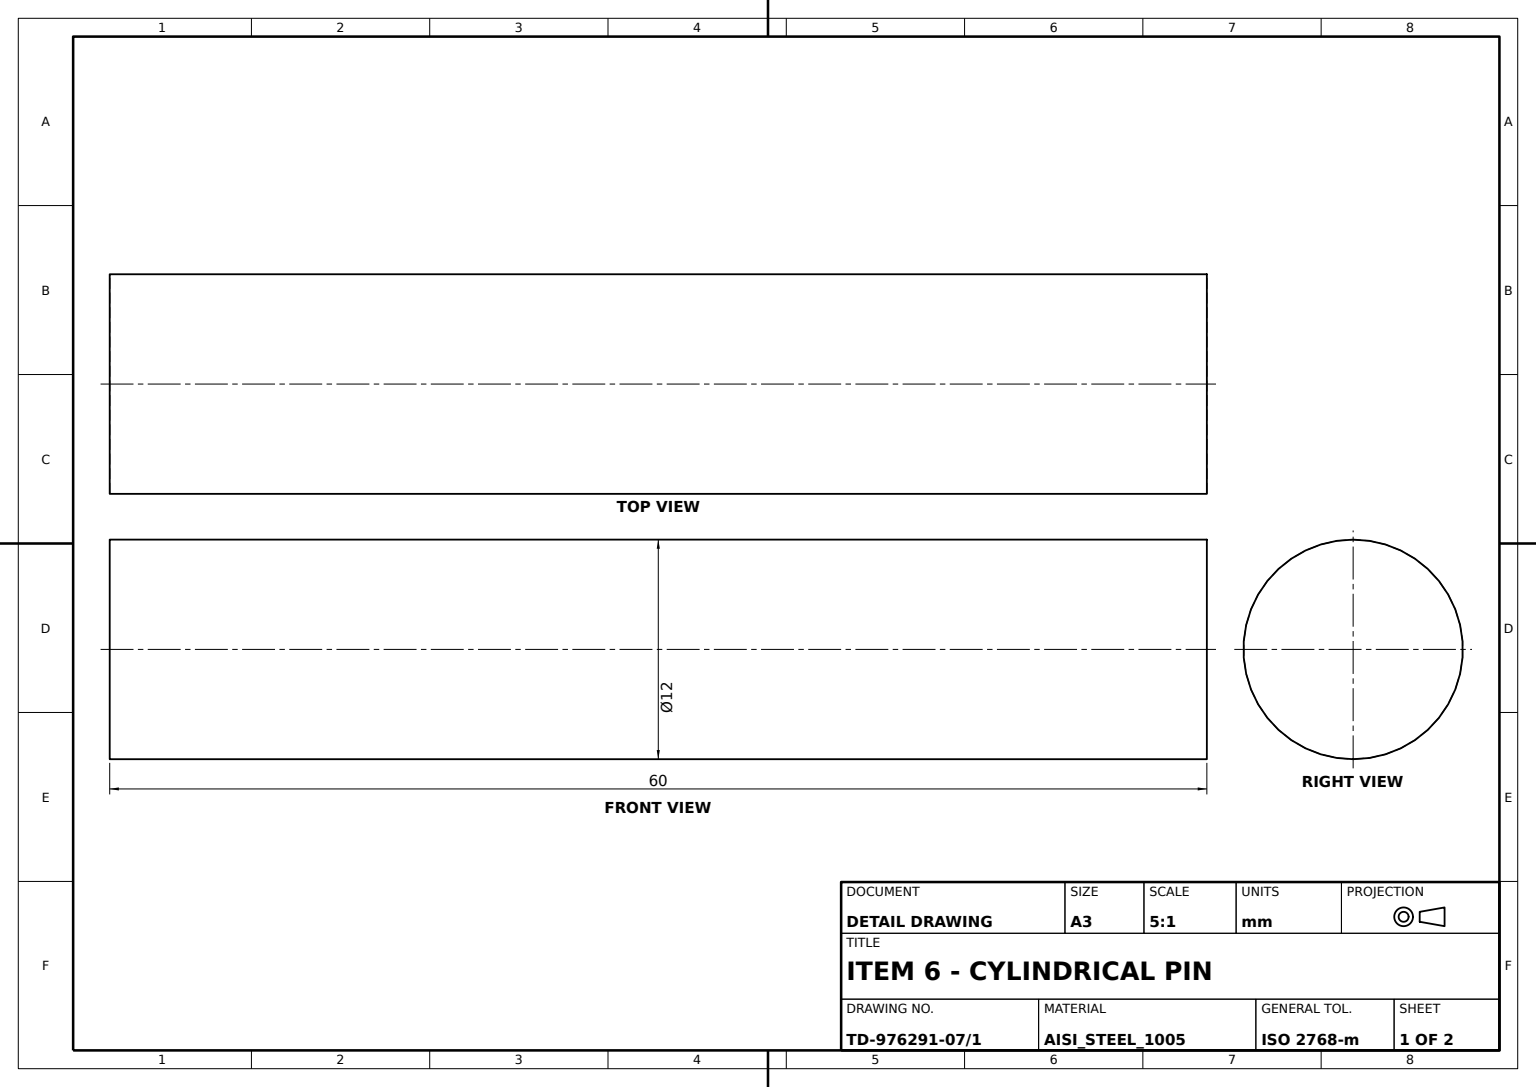
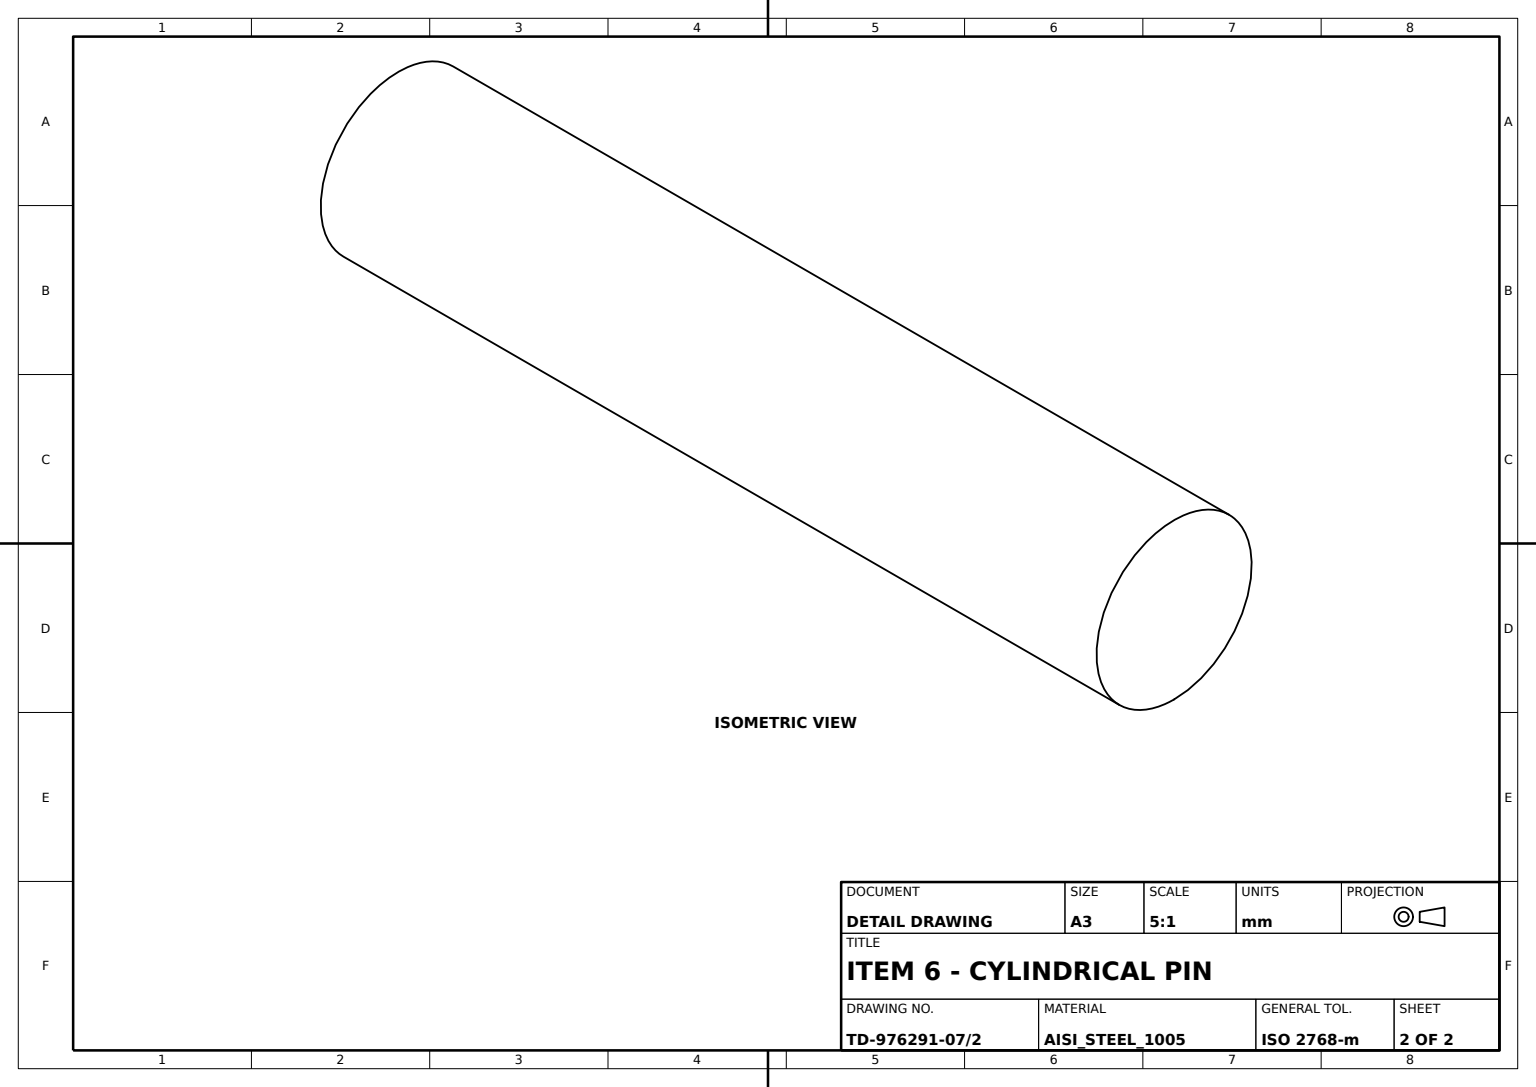
ISO-10303-21;
HEADER;
FILE_DESCRIPTION((''),'2;1');
FILE_NAME('','',(''),(''),'','','');
FILE_SCHEMA(('AUTOMOTIVE_DESIGN'));
ENDSEC;
DATA;
#1=APPLICATION_CONTEXT('');
#2=PRODUCT_CONTEXT('',#1,'mechanical');
#3=PRODUCT('','','',(#2));
#4=PRODUCT_DEFINITION_FORMATION('','',#3);
#5=PRODUCT_DEFINITION_CONTEXT('',#1,'design');
#6=PRODUCT_DEFINITION('','',#4,#5);
#7=PRODUCT_DEFINITION_SHAPE('','',#6);
#8=(LENGTH_UNIT()NAMED_UNIT(*)SI_UNIT(.MILLI.,.METRE.));
#9=(NAMED_UNIT(*)PLANE_ANGLE_UNIT()SI_UNIT($,.RADIAN.));
#10=(NAMED_UNIT(*)SI_UNIT($,.STERADIAN.)SOLID_ANGLE_UNIT());
#11=UNCERTAINTY_MEASURE_WITH_UNIT(LENGTH_MEASURE(0.005),#8,'distance_accuracy_value','');
#12=(GEOMETRIC_REPRESENTATION_CONTEXT(3)GLOBAL_UNCERTAINTY_ASSIGNED_CONTEXT((#11))GLOBAL_UNIT_ASSIGNED_CONTEXT((#8,#9,#10))REPRESENTATION_CONTEXT('',''));
#13=CARTESIAN_POINT('',(6.,0.,-30.));
#14=VERTEX_POINT('',#13);
#15=CARTESIAN_POINT('',(0.,0.,-30.));
#16=DIRECTION('',(0.,0.,1.));
#17=DIRECTION('',(1.,0.,0.));
#18=AXIS2_PLACEMENT_3D('',#15,#16,#17);
#19=CIRCLE('',#18,6.);
#20=EDGE_CURVE('',#14,#14,#19,.T.);
#21=ORIENTED_EDGE('',*,*,#20,.F.);
#22=EDGE_LOOP('',(#21));
#23=FACE_BOUND('',#22,.T.);
#24=PLANE('',#18);
#25=ADVANCED_FACE('',(#23),#24,.F.);
#26=CARTESIAN_POINT('',(6.,0.,30.));
#27=VERTEX_POINT('',#26);
#28=CARTESIAN_POINT('',(0.,0.,30.));
#29=AXIS2_PLACEMENT_3D('',#28,#16,#17);
#30=CIRCLE('',#29,6.);
#31=EDGE_CURVE('',#27,#27,#30,.T.);
#32=ORIENTED_EDGE('',*,*,#31,.T.);
#33=EDGE_LOOP('',(#32));
#34=FACE_BOUND('',#33,.T.);
#35=PLANE('',#29);
#36=ADVANCED_FACE('',(#34),#35,.T.);
#37=ORIENTED_EDGE('',*,*,#20,.T.);
#38=EDGE_LOOP('',(#37));
#39=FACE_BOUND('',#38,.T.);
#40=ORIENTED_EDGE('',*,*,#31,.F.);
#41=EDGE_LOOP('',(#40));
#42=FACE_BOUND('',#41,.T.);
#43=DIRECTION('',(0.,0.,-1.));
#44=DIRECTION('',(-1.,0.,0.));
#45=AXIS2_PLACEMENT_3D('',#28,#43,#44);
#46=CYLINDRICAL_SURFACE('',#45,6.);
#47=ADVANCED_FACE('',(#39,#42),#46,.T.);
#48=CLOSED_SHELL('',(#25,#36,#47));
#49=MANIFOLD_SOLID_BREP('',#48);
#50=ADVANCED_BREP_SHAPE_REPRESENTATION('',(#49),#12);
#51=SHAPE_DEFINITION_REPRESENTATION(#7,#50);
ENDSEC;
END-ISO-10303-21;
